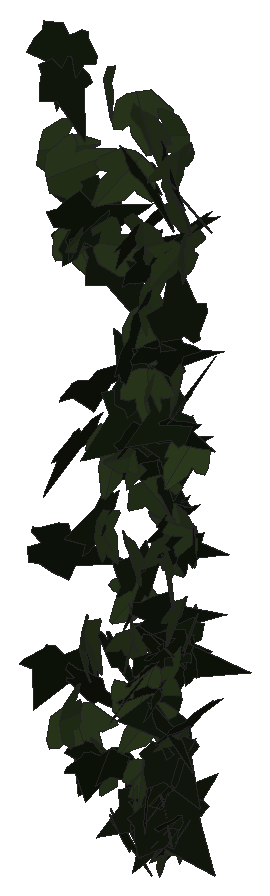
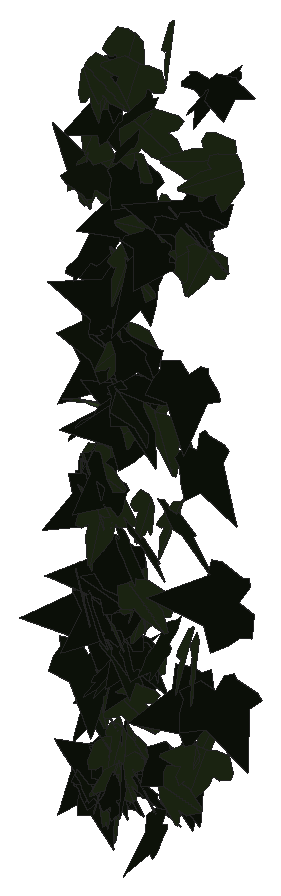
# SketchUp Ruby script. Lengths in inches.
U = 1.inch
M = Sketchup.active_model
def pt(a) = Geom::Point3d.new(a.map { |v| v * U })
def face(e, loops, mat)
  f = e.add_face(loops[0].map { |a| pt(a) })
  loops[1..].each { |l| e.add_face(l.map { |a| pt(a) }).erase! }
  f.material = f.back_material = mat if mat
  f
end
# faces: each face lists its corners as indices into pts; further lists are holes
def faces(e, pts, list, mat = nil) = list.each { |f| face(e, (f[0].is_a?(Array) ? f : [f]).map { |l| l.map { |i| pts[i] } }, mat) }
# xy, xz, yz: faces in a plane at the given z, y or x. An outline is a flat list of corners, or four numbers for a rectangle; further outlines are holes
def ring(l) = l.size == 4 ? [[l[0], l[1]], [l[2], l[1]], [l[2], l[3]], [l[0], l[3]]] : l.each_slice(2).to_a
def flat(e, list, mat, &to3) = list.each { |f| face(e, (f[0].is_a?(Array) ? f : [f]).map { |l| ring(l).map { |u, v| to3.(u, v) } }, mat) }
def xy(e, z, list, mat = nil) = flat(e, list, mat) { |x, y| [x, y, z] }
def xz(e, y, list, mat = nil) = flat(e, list, mat) { |x, z| [x, y, z] }
def yz(e, x, list, mat = nil) = flat(e, list, mat) { |y, z| [x, y, z] }
def lines(e, pts, list) = list.each { |a, b| e.add_line(pt(pts[a]), pt(pts[b])) }
# prism: a flat outline (further loops are holes) pulled along v
def prism(e, loops, v, mat = nil)
  f = face(e, loops, mat); d = Geom::Vector3d.new(v.map { |x| x * U })
  f.pushpull(f.normal.samedirection?(d) ? d.length : -d.length)
end
def box(e, o, s, mat = nil) = prism(e, [[o, [o[0] + s[0], o[1], o[2]], [o[0] + s[0], o[1] + s[1], o[2]], [o[0], o[1] + s[1], o[2]]]], [0, 0, s[2]], mat)
def at(x, y, z, deg = 0) = Geom::Transformation.translation(pt([x, y, z])) * Geom::Transformation.rotation(ORIGIN, Z_AXIS, deg.degrees)
def axes(o, x, y, z) = Geom::Transformation.new([*x, 0, *y, 0, *z, 0, *pt(o).to_a, 1])
def part(name) = M.definitions.add(name)
# library, detail: a bought-in or finely detailed component or shape, given as its bounding box
def library(name, o, s) = part(name).tap { |d| box(d.entities, o, s) }
def detail(e, o, s) = box(e.add_group.entities, o, s)
def put(e, d, t, mat = nil) = e.add_instance(d, t).tap { |i| i.material = mat if mat }
def group(e, t, mat = nil) = e.add_group.tap { |g| g.transformation = t; g.material = mat if mat }.entities
root = M.entities
M.materials.add("efeu1").color = [18, 25, 13]
M.materials.add("efeu2").color = [43, 57, 29]
c1 = part("ivyleaf_10")
p = [[0,0.5,-0.03],[-0.0625,2.02,-0.43],[-0.19,2.01,-0.46],[-0.54,1.05,-0.29],[-0.52,0.625,-0.18],[-0.83,0.76,-0.28],
  [-1.16,0.64,-0.33],[-1.15,0.33,-0.24],[-0.77,-0.39,0.02],[-0.3,-0.51,0.16],[0.04,-0.48,0.23],[-0.02,2.01,-0.4375],
  [-0.06,2.01,-0.43],[0.04,-0.49,0.23],[0.67,-0.49,0.14],[1.38,0.36,-0.2],[1.375,0.51,-0.24],[0.81,0.65,-0.19],
  [0.62,0.59,-0.15],[0.6,1.09,-0.28],[0.5,1.23,-0.31]]
faces(c1.entities,p,[[0,1,2,3,4,5,6,7,8,9,10],[11,12,0,13,14,15,16,17,18,19,20]],"efeu2")
c2 = part("ivyleaf_9")
p = [[1.54,2.16,1.25],[1.36,2.04,1.19],[-0.21,0.99,0.68],[-0.71,1.11,0.82],[-0.85,0.86,0.67],[-0.8,0.17,0.21],
  [-0.9,-0.01,0.1],[-0.67,-0.16,-0.02],[-0.08,-0.08,-0.05],[-0.03,-0.6,-0.4],[0.65,-0.88,-0.66],[0.83,-0.6,-0.49],
  [1.29,-0.42,-0.43],[1.8125,-0.07,-0.26],[1.21,0.44,0.15]]
faces(c2.entities,p,[[0,1,2,3,4,5,6,7,8,9,10,11,12,13,14]],"efeu1")
put(root,c1,axes([584.76,127.25,224.19],[-0.73947,-0.41748,-0.54081],[0.52248,0.16793,-0.84404],[0.44021,-0.9006,0.09331]))
put(root,c1,axes([584.02,126.86,216.98],[0.28064,-0.54548,-1.0018],[-0.39757,0.9202,-0.61243],[1.06915,0.48536,0.03522]))
put(root,c1,axes([583.87,127.64,210.08],[0.79924,-0.25023,0.2347],[0.22141,-0.07828,-0.83746],[0.26206,0.8293,-0.00823]))
put(root,c1,axes([583.58,128.27,224.96],[-0.20325,-0.16526,-1.05917],[-0.41797,-0.9805,0.23319],[-0.98714,0.44919,0.11934]))
put(root,c2,axes([585.74,127.95,227.87],[-0.80139,-0.31932,0.32751],[-0.30184,-0.12723,-0.86264],[0.34368,-0.85633,0.00605]))
put(root,c2,axes([585.4,127,231.27],[0.55219,0.84737,-0.15856],[-0.1014,-0.12315,-1.01125],[-0.85609,0.56115,0.01751]))
put(root,c1,axes([582.56,127.13,242.96],[-0.4836,0.77232,0.43098],[-0.37968,0.26234,-0.89616],[-0.79879,-0.59227,0.16504]))
put(root,c2,axes([585.1,127.83,208.76],[-0.71015,-0.37966,-0.20513],[0.1991,0.06219,-0.80438],[0.38286,-0.73656,0.03782]))
put(root,c2,axes([585.07,127.82,208.02],[-0.86125,-0.16297,-0.22566],[0.2288,0.00345,-0.87571],[0.15853,-0.89032,0.03791]))
put(root,c2,axes([585.78,127.72,211.22],[-0.80128,0.2027,-0.295],[0.281,-0.09175,-0.82631],[-0.22169,-0.84892,0.01887]))
put(root,c2,axes([585.58,127.34,211.82],[0.17833,-0.73875,-0.70748],[-0.12345,0.69735,-0.7593],[1.0154,0.21452,0.03194]))
put(root,c1,axes([583.6875,127.5,230.92],[0.74618,-0.33143,-0.64862],[0.66427,-0.0713,0.80062],[-0.29882,-0.9861,0.16011]))
put(root,c1,axes([585.78,127.9,235.62],[-0.44766,-0.63142,0.56987],[-0.31501,-0.47511,-0.77388],[0.79007,-0.5472,0.01434]))
put(root,c1,axes([585.01,127.38,207.53],[-0.39783,-0.26488,-0.67516],[0.67866,0.13561,-0.4531],[0.25578,-0.77183,0.15209]))
put(root,c1,axes([583.49,127.49,220.9375],[-0.74685,0.47621,-0.13034],[0.08483,-0.10906,-0.88457],[-0.48638,-0.75025,0.04585]))
put(root,c2,axes([583.9,127.72,214.375],[-0.49359,0.53578,-0.45611],[0.21714,-0.41397,-0.72126],[-0.66929,-0.52943,0.10238]))
put(root,c1,axes([584.4375,127.42,241.875],[-1.05117,0.32669,-0.05232],[0.04859,-0.01995,-1.10075],[-0.32726,-1.05228,0.00462]))
put(root,c1,axes([585,127.49,210.02],[-0.45396,0.7013,-0.08952],[0.0575,-0.0694,-0.83534],[-0.70465,-0.45747,-0.0105]))
put(root,c1,axes([585.83,127.86,218.57],[0.19381,-0.82248,0.23049],[0.07254,-0.21965,-0.84478],[0.85108,0.20602,0.01951]))
put(root,c2,axes([583.72,127.74,208.08],[-0.80747,0.14154,0.11643],[-0.1107,0.04253,-0.81947],[-0.14606,-0.81471,-0.02255]))
put(root,c1,axes([584.27,127.48,236.53],[-0.9506,0.11126,0.1656],[-0.16689,-0.0017,-0.95686],[-0.10931,-0.96491,0.02078]))
put(root,c1,axes([583.98,127.3,213.16],[0.95658,0.53186,-0.42665],[0.37381,0.20567,1.0945],[0.57024,-1.02702,-0.00177]))
put(root,c2,axes([584.66,127.95,240.32],[0.09519,0.02377,-1.09498],[1.09518,-0.01319,0.09492],[-0.01108,-1.09903,-0.02482]))
put(root,c2,axes([585.01,127.89,212.96],[0.5435,-0.74722,0.19315],[0.1554,-0.12545,-0.92258],[0.75598,0.563,0.05078]))
put(root,c1,axes([583.55,127.49,216.61],[-0.48373,-0.68264,-0.27146],[0.15698,0.22147,-0.83665],[0.71766,-0.50857,0.00004]))
put(root,c1,axes([584.15,127.7,228.98],[1.00356,0.14723,0.24905],[0.24264,0.06135,-1.014],[-0.15757,1.03218,0.02474]))
put(root,c2,axes([585.06,128.57,212.84],[0.25107,-0.87021,-0.69907],[0.20085,-0.66962,0.90568],[-1.09801,-0.32147,0.00582]))
put(root,c1,axes([585.86,127.77,229.67],[0.61574,-0.69752,-0.06592],[-0.01681,0.07302,-0.92973],[0.70042,0.61494,0.03563]))
put(root,c2,axes([581.83,127.53,210.04],[0.18182,0.90738,-0.5233],[-0.09683,-0.51429,-0.92541],[-1.04298,0.20593,-0.00532]))
put(root,c2,axes([581.77,127.63,210.13],[0.40166,0.55414,-0.77223],[-0.48205,-0.60377,-0.68398],[-0.81917,0.627,0.02385]))
put(root,c1,axes([585.04,128.01,220.28],[-0.44675,0.5405,-0.70029],[0.37654,-0.59372,-0.69847],[-0.80048,-0.58094,0.06228]))
put(root,c1,axes([582.41,127.85,225.35],[1.24608,-0.24335,-0.01156],[-0.00775,0.02061,-1.26949],[0.2435,1.24597,0.01874]))
put(root,c1,axes([585.78,127.79,240.3],[-0.12324,-1.0959,-0.05158],[0.00564,0.05127,-1.10281],[1.0971,-0.12337,-0.00013]))
put(root,c2,axes([585.41,127.39,208.71],[-0.12827,-0.55305,-1.09213],[0.24879,1.06342,-0.56773],[1.19863,-0.27991,0.00096]))
put(root,c2,axes([583.52,128.43,226.78],[-0.90719,-0.51318,0.4194],[-0.33398,-0.26011,-1.0407],[0.57246,-0.96501,0.05748]))
put(root,c1,axes([580.5,126.97,211.62],[-0.07116,0.30882,1.05388],[-0.54394,0.90754,-0.30266],[-0.95403,-0.54047,0.09396]))
put(root,c2,axes([585.74,128.03,208.04],[-0.32988,0.43612,-0.60827],[0.01887,-0.65967,-0.48321],[-0.74822,-0.20892,0.25599]))
put(root,c1,axes([585.64,127.9,212.04],[-0.10925,-0.86601,0.07229],[-0.00941,-0.07168,-0.87287],[0.86897,-0.10965,-0.00036]))
put(root,c2,axes([584.17,126.72,231.58],[-0.17438,0.30916,-1.40001],[-1.05244,0.93014,0.33649],[0.97364,1.06079,0.11297]))
put(root,c2,axes([584.82,127.73,214.23],[-0.71333,0.6134,-0.0597],[0.04438,-0.03996,-0.9408],[-0.6147,-0.71471,0.00136]))
put(root,c1,axes([585.11,127.93,206.85],[0.15864,-0.809,0.01458],[0.0118,-0.01255,-0.82436],[0.80905,0.15882,0.00916]))
put(root,c1,axes([583.09,128.1,238.84],[0.79727,0.46343,-0.72744],[-0.66397,-0.30253,-0.92043],[-0.55053,1.036,0.05662]))
put(root,c1,axes([582.05,127.44,221.1875],[-0.27212,0.86418,0.41282],[-0.15034,0.38529,-0.90566],[-0.94584,-0.30986,0.02519]))
put(root,c1,axes([580,127.11,237.98],[0.12246,0.14154,-1.2266],[0.85623,0.87837,0.18684],[0.88963,-0.86487,-0.01099]))
put(root,c2,axes([583.32,128.27,238.83],[0.66856,-0.85836,0.42256],[0.28596,-0.31266,-1.08756],[0.91299,0.72648,0.0312]))
put(root,c2,axes([584.86,127.88,239.15],[0.97723,-0.45896,0.17866],[0.15881,-0.08213,-1.07962],[0.46621,0.99003,-0.00674]))
put(root,c2,axes([579.48,127.95,213.89],[0.26813,0.78463,-0.83477],[-0.27638,-0.7877,-0.82916],[-1.1118,0.38504,0.0048]))
put(root,c2,axes([583.87,127.375,213.6875],[0.55687,0.6644,0.17345],[0.11289,0.1317,-0.8669],[-0.67732,0.56819,-0.00188]))
put(root,c1,axes([583.93,127.84,208.93],[-0.03352,0.83117,0.01201],[0.01205,0.01251,-0.83176],[-0.83117,-0.03334,-0.01254]))
put(root,c2,axes([585.21,127.52,224.76],[0.56715,-0.17976,-0.69313],[-0.55595,0.44673,-0.57075],[0.4513,0.77622,0.16796]))
put(root,c1,axes([581.34,127.51,215.5],[-0.49827,0.819,0.47792],[-0.29378,0.37999,-0.95746],[-0.90158,-0.57645,0.04786]))
put(root,c2,axes([583.84,127.92,236.36],[-0.38441,0.96493,-0.38312],[0.11293,-0.36726,-1.03827],[-1.03205,-0.3996,0.0291]))
put(root,c2,axes([579.29,128.17,242.09],[0.29132,-0.97442,-0.31232],[-0.07431,0.30373,-1.01693],[1.02055,0.30027,0.0151]))
put(root,c2,axes([580.22,128.17,224.82],[-0.51238,0.86042,-0.66356],[0.32061,-0.58125,-1.00126],[-1.03819,-0.60415,0.01828]))
put(root,c2,axes([581.94,128.09,215.35],[0.77454,-0.68046,-0.05949],[-0.04455,0.03942,-1.031],[0.68161,0.77582,0.00021]))
put(root,c2,axes([583.68,127.65,219.49],[-0.37667,0.62704,0.50206],[-0.32978,0.38492,-0.72815],[-0.73245,-0.49576,0.06966]))
put(root,c1,axes([581.04,127.43,214.97],[-0.37115,0.4365,0.95103],[-0.71899,0.62678,-0.56827],[-0.76029,-0.80582,0.07314]))
put(root,c1,axes([585.89,128,237.17],[-0.9342,0.45604,-0.30383],[-0.27396,0.13138,1.03957],[0.47458,0.97354,0.00203]))
put(root,c2,axes([581.72,127.86,221.35],[-0.76336,0.75691,0.20636],[-0.15072,0.14107,-1.07498],[-0.76992,-0.77807,0.00584]))
put(root,c2,axes([583.875,127.88,216.43],[0.86931,-0.10983,0.25876],[0.25632,-0.03561,-0.87622],[0.11542,0.90631,-0.00307]))
put(root,c2,axes([584.61,127.33,209.53],[-0.02149,0.15908,-1.25961],[-1.15379,0.52326,0.08577],[0.52981,1.14599,0.13569]))
put(root,c1,axes([585.43,127.98,207.82],[-0.24217,0.78573,-0.02934],[0.00799,-0.02824,-0.8222],[-0.78624,-0.2423,0.00068]))
put(root,c2,axes([580.36,127.94,213.07],[1.02947,-0.21255,0.50691],[0.4977,-0.09638,-1.05116],[0.23332,1.14345,0.00563]))
put(root,c2,axes([583.8,127.99,226.26],[-0.33838,0.96626,-0.33618],[0.1306,-0.31039,-1.02361],[-1.0147,-0.36218,-0.01964]))
put(root,c1,axes([583.88,128.36,212.34],[0.76778,0.34522,-0.56232],[-0.52186,-0.21025,-0.84161],[-0.40378,0.92816,0.0185]))
put(root,c2,axes([585.24,127.625,227.1],[0.7833,0.42161,0.25822],[0.22634,0.12431,-0.88955],[-0.43955,0.81534,0.0021]))
put(root,c2,axes([585.09,127.93,209.04],[-0.36576,0.82628,-0.11014],[0.05888,-0.09437,-0.90348],[-0.83151,-0.37014,-0.01552]))
put(root,c2,axes([585.96,128.3,208.125],[-0.58692,0.44817,-0.34999],[0.23533,-0.26646,-0.73583],[-0.51766,-0.62926,0.06231]))
put(root,c2,axes([585.88,128.01,211.15],[-0.50679,0.66469,0.00477],[-0.00098,0.00525,-0.83585],[-0.66471,-0.50679,-0.0024]))
put(root,c1,axes([585.59,128.875,225.64],[-1.00041,-0.06556,0.05139],[0.04884,-0.96328,-0.2783],[0.06748,-0.27484,0.96315]))
put(root,c1,axes([584.5,128.3,214.7],[0.83507,-0.44126,-0.51034],[0.45056,-0.23968,0.94449],[-0.50215,-0.94887,-0.00125]))
put(root,c2,axes([582.34,128.04,206.83],[0.8405,-0.39894,-0.28251],[-0.25222,0.12744,-0.93034],[0.41874,0.8775,0.00668]))
put(root,c2,axes([585.6,128.04,207.21],[-0.21715,0.76312,-0.18302],[0.02461,-0.18318,-0.793],[-0.78437,-0.21702,0.02579]))
put(root,c2,axes([583.65,127.79,225.44],[0.09829,-0.1377,0.9487],[0.89969,0.34252,-0.0435],[-0.33098,0.89016,0.1635]))
put(root,c2,axes([581.07,127.83,227.89],[0.22643,1.03608,-0.15869],[-0.04185,-0.15328,-1.06051],[-1.04733,0.23012,0.00806]))
put(root,c2,axes([583.78,127.79,208.49],[-0.65871,0.19108,-0.76987],[-0.75448,0.15802,0.68477],[0.24489,1.00082,0.03887]))
put(root,c2,axes([583.88,128.54,219.57],[-0.84163,0.40254,-0.59563],[0.54113,-0.24901,-0.93291],[-0.47328,-1.00055,-0.00745]))
put(root,c2,axes([584.41,127.99,230.05],[0.49382,-0.2541,0.89898],[0.9331,0.18371,-0.46063],[-0.04552,1.0091,0.31023]))
put(root,c2,axes([584.08,128.92,207.62],[0.00618,0.01942,0.89607],[-0.46436,-0.76638,0.01981],[0.76661,-0.46438,0.00477]))
put(root,c1,axes([585.8,128.13,222.36],[0.19,-0.04214,-1.01888],[-0.93505,0.40637,-0.19117],[0.40692,0.95346,0.03645]))
put(root,c2,axes([584.28,127.77,217.51],[0.61574,0.12702,0.93636],[0.89438,0.28231,-0.62643],[-0.30493,1.08453,0.0534]))
put(root,c1,axes([586,128.25,236.17],[-0.16465,0.94757,0.00833],[-0.28644,-0.04171,-0.91721],[-0.90327,-0.1595,0.28934]))
put(root,c2,axes([580.17,127.82,234.98],[0.31891,0.01601,1.17296],[1.14634,0.25372,-0.31514],[-0.24896,1.18876,0.05146]))
put(root,c2,axes([583.57,128.05,228.25],[-0.95327,0.12467,-0.46681],[-0.47869,-0.10337,0.94993],[0.06566,1.05639,0.14804]))
put(root,c1,axes([584.47,128.4,209.84],[-0.57406,-0.75332,0.01209],[-0.00586,-0.01074,-0.94712],[0.75339,-0.57409,0.00185]))
put(root,c2,axes([585.76,128.16,231.8],[-0.46701,-0.81019,0.7348],[0.36512,0.63767,0.93514],[-1.03103,0.5928,-0.00167]))
put(root,c1,axes([583.91,128.57,209.15],[0.40346,0.86539,-0.34236],[-0.16356,-0.3014,-0.95461],[-0.91616,0.4349,0.01965]))
put(root,c2,axes([583.875,127.73,214.59],[0.3022,0.70283,0.39989],[0.07949,0.39901,-0.76137],[-0.80471,0.30335,0.07497]))
put(root,c1,axes([580.27,129.1875,234.56],[-0.0581,0.15609,-1.05329],[-0.15538,-1.04481,-0.14626],[-1.0534,0.1455,0.07966]))
put(root,c1,axes([579.92,128.26,210.875],[0.90307,0.704,0.37846],[0.29225,0.24066,-1.14501],[-0.74393,0.94913,0.00961]))
put(root,c2,axes([585.36,128.08,208.46],[-0.08156,-0.07797,0.83364],[0.78666,0.27967,0.10313],[-0.2867,0.78955,0.0458]))
put(root,c2,axes([581.9375,128.48,234.03],[-0.43183,-0.50123,-0.85511],[0.54056,0.66273,-0.66145],[0.83081,-0.69173,-0.0141]))
put(root,c2,axes([586.19,127.89,213.16],[-0.01956,1.17847,0.10768],[-0.12527,0.10502,-1.1722],[-1.17673,-0.03077,0.123]))
put(root,c2,axes([585.58,127.71,227.79],[-0.48656,0.93318,-0.35456],[-0.16093,0.31595,1.05241],[0.98521,0.51247,-0.0032]))
put(root,c2,axes([585.68,128.57,216.47],[-0.44919,0.11465,0.8004],[-0.7674,0.22802,-0.46333],[-0.25474,-0.88906,-0.01561]))
put(root,c1,axes([581.65,128.19,234.48],[-0.0556,-0.14219,1.15468],[0.9822,0.61382,0.12288],[-0.62353,0.97959,0.09061]))
put(root,c1,axes([584,128.02,232.74],[-0.22297,0.88829,0.58408],[-0.27125,0.5295,-0.90884],[-1.02793,-0.33241,0.11313]))
put(root,c2,axes([584.54,127.89,215.84],[0.36749,0.48672,-1.25283],[0.68711,1.04824,0.60878],[1.15515,-0.77836,0.03645]))
put(root,c2,axes([580.6,127.97,234.54],[-1.09258,0.39548,-0.34808],[-0.33263,0.10364,1.16186],[0.40856,1.142,0.0151]))
put(root,c1,axes([583.08,128.51,241.64],[0.91922,0.45637,0.34547],[0.2949,0.18256,-1.02582],[-0.49057,0.96488,0.03068]))
put(root,c2,axes([585.98,128.2,220.86],[0.03913,-0.04296,1.00588],[-0.4237,0.91246,0.05546],[-0.9133,-0.42515,0.01737]))
put(root,c2,axes([583.79,127.74,234.67],[-0.12752,0.68715,-0.86321],[-0.28353,0.81936,0.69414],[1.06626,0.30006,0.08134]))
put(root,c1,axes([579.67,128.46,234.18],[0.70768,0.57922,0.41777],[0.28707,0.30781,-0.91306],[-0.65392,0.76197,0.05128]))
put(root,c1,axes([584.41,127.93,228.2],[-0.00347,-0.06408,1.04411],[-0.39632,0.96636,0.05799],[-0.96809,-0.39538,-0.02748]))
put(root,c1,axes([581.51,128.43,209.03],[0.06918,0.05614,-1.07073],[-0.93808,0.52278,-0.0332],[0.51924,0.93699,0.08268]))
put(root,c2,axes([583.52,128.96,229.07],[-0.68523,-0.28473,-0.77919],[0.71932,0.29953,-0.74203],[0.41327,-0.99346,-0.0004]))
put(root,c1,axes([584.14,128.55,210.45],[-0.83861,0.52478,0.10631],[-0.08765,0.06033,-0.98926],[-0.52821,-0.84317,-0.00462]))
put(root,c1,axes([578.72,128.08,238.24],[-0.08367,-0.13791,-1.07502],[0.71897,0.79977,-0.15856],[0.81103,-0.72322,0.02966]))
put(root,c2,axes([584.65,129.39,225.58],[-0.12289,-1.06042,0.18662],[-0.0195,-0.18561,-1.06752],[1.07654,-0.12441,0.00197]))
put(root,c2,axes([584.22,128.15,214.06],[-0.1319,0.75013,0.61345],[-0.29519,0.55857,-0.7465],[-0.92297,-0.28585,0.15109]))
put(root,c2,axes([585.95,128.49,216.17],[-0.1383,0.08305,-0.89826],[-0.90138,-0.04877,0.13428],[-0.03578,0.90753,0.08942]))
put(root,c1,axes([585.18,128.61,240.89],[0.45254,-0.17952,-0.95605],[-0.86732,0.40298,-0.48622],[0.44046,0.97797,0.02486]))
put(root,c1,axes([582.86,128.88,217.85],[0.86574,0.05651,-0.53903],[-0.54056,0.01628,-0.86648],[-0.03934,1.01971,0.04371]))
put(root,c1,axes([585.38,128.87,221.3125],[0.86739,-0.3633,-0.20555],[-0.18557,0.08899,-0.94035],[0.3739,0.88696,0.01015]))
put(root,c1,axes([585.77,128.87,217.39],[0.49912,-0.83859,-0.11866],[-0.06102,0.10177,-0.97588],[0.84474,0.50283,-0.00039]))
put(root,c2,axes([580.35,129.3125,236.06],[-0.79191,-0.69283,-0.12966],[0.10431,0.07767,-1.05216],[0.69709,-0.79869,0.01015]))
put(root,c2,axes([585.04,128.97,235.86],[0.36428,-0.96527,0.23963],[0.97488,0.39708,0.11752],[-0.19694,0.18014,1.025]))
put(root,c2,axes([583.68,128.11,225.71],[-0.69558,0.62419,-0.48584],[-0.35786,0.32863,0.93457],[0.7054,0.78222,-0.00495]))
put(root,c2,axes([584.77,128,222.01],[0.27757,0.62392,0.73487],[0.23064,0.69954,-0.68103],[-0.93601,0.35739,0.05011]))
put(root,c2,axes([583.52,127.98,225.07],[0.17584,0.68573,-0.90844],[0.02881,0.91624,0.69719],[1.13783,-0.12917,0.12274]))
put(root,c2,axes([578.21,128.37,218.75],[0.41403,0.46794,-1.0981],[0.73858,0.81263,0.62477],[0.93771,-0.84668,-0.00725]))
put(root,c2,axes([578.76,129.21,243.03],[-0.71542,-0.61995,-0.43145],[0.35045,0.25397,-0.94604],[0.66908,-0.79591,0.03419]))
put(root,c2,axes([584.77,128.13,215.97],[0.58402,0.61328,0.46857],[0.24669,0.40844,-0.84206],[-0.73131,0.62754,0.09014]))
put(root,c2,axes([585.2,128.25,220.99],[0.61638,0.43623,0.52631],[0.42944,0.30427,-0.75513],[-0.53186,0.75122,0.00023]))
put(root,c1,axes([584.71,128.6875,221.05],[-0.36547,-1.03448,-0.4204],[0.18258,0.38103,-1.09633],[1.10161,-0.40635,0.04223]))
